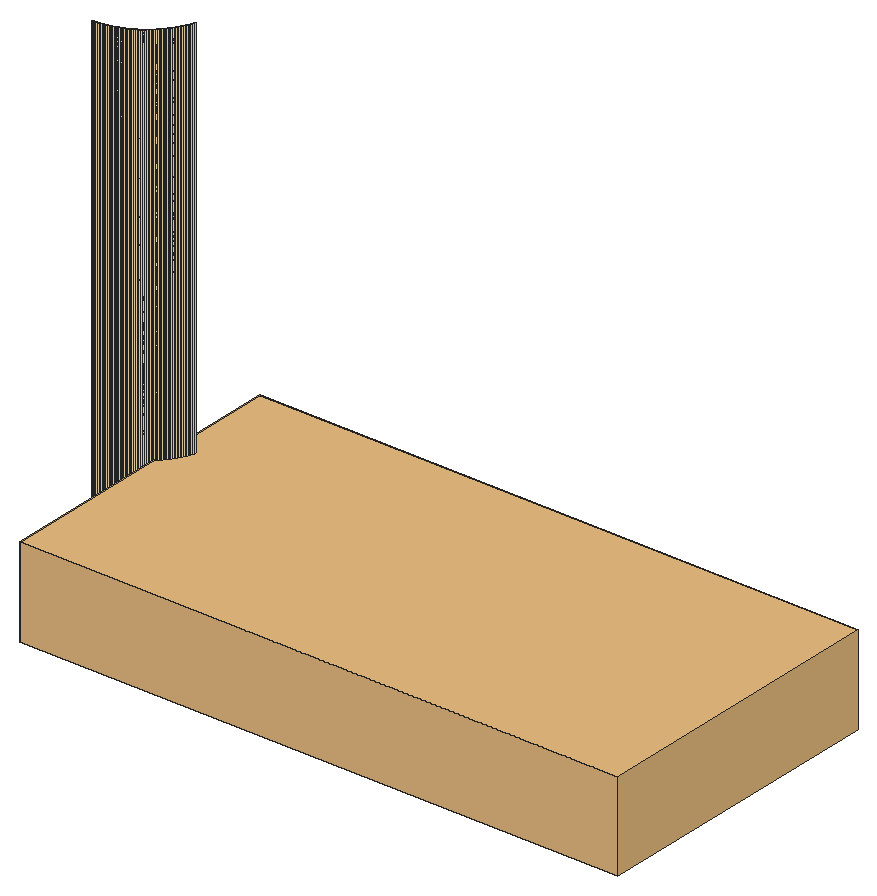
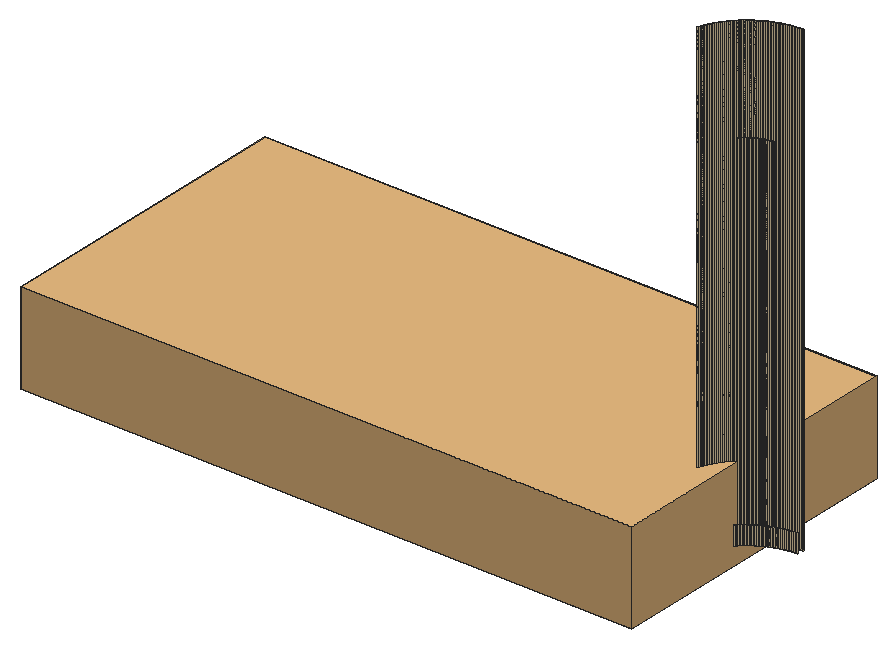
# SketchUp Ruby script. Lengths in inches.
U = 1.inch
M = Sketchup.active_model
def pt(a) = Geom::Point3d.new(a.map { |v| v * U })
def face(e, loops, mat)
  f = e.add_face(loops[0].map { |a| pt(a) })
  loops[1..].each { |l| e.add_face(l.map { |a| pt(a) }).erase! }
  f.material = f.back_material = mat if mat
  f
end
# faces: each face lists its corners as indices into pts; further lists are holes
def faces(e, pts, list, mat = nil) = list.each { |f| face(e, (f[0].is_a?(Array) ? f : [f]).map { |l| l.map { |i| pts[i] } }, mat) }
# xy, xz, yz: faces in a plane at the given z, y or x. An outline is a flat list of corners, or four numbers for a rectangle; further outlines are holes
def ring(l) = l.size == 4 ? [[l[0], l[1]], [l[2], l[1]], [l[2], l[3]], [l[0], l[3]]] : l.each_slice(2).to_a
def flat(e, list, mat, &to3) = list.each { |f| face(e, (f[0].is_a?(Array) ? f : [f]).map { |l| ring(l).map { |u, v| to3.(u, v) } }, mat) }
def xy(e, z, list, mat = nil) = flat(e, list, mat) { |x, y| [x, y, z] }
def xz(e, y, list, mat = nil) = flat(e, list, mat) { |x, z| [x, y, z] }
def yz(e, x, list, mat = nil) = flat(e, list, mat) { |y, z| [x, y, z] }
def lines(e, pts, list) = list.each { |a, b| e.add_line(pt(pts[a]), pt(pts[b])) }
# prism: a flat outline (further loops are holes) pulled along v
def prism(e, loops, v, mat = nil)
  f = face(e, loops, mat); d = Geom::Vector3d.new(v.map { |x| x * U })
  f.pushpull(f.normal.samedirection?(d) ? d.length : -d.length)
end
def box(e, o, s, mat = nil) = prism(e, [[o, [o[0] + s[0], o[1], o[2]], [o[0] + s[0], o[1] + s[1], o[2]], [o[0], o[1] + s[1], o[2]]]], [0, 0, s[2]], mat)
def at(x, y, z, deg = 0) = Geom::Transformation.translation(pt([x, y, z])) * Geom::Transformation.rotation(ORIGIN, Z_AXIS, deg.degrees)
def axes(o, x, y, z) = Geom::Transformation.new([*x, 0, *y, 0, *z, 0, *pt(o).to_a, 1])
def part(name) = M.definitions.add(name)
# library, detail: a bought-in or finely detailed component or shape, given as its bounding box
def library(name, o, s) = part(name).tap { |d| box(d.entities, o, s) }
def detail(e, o, s) = box(e.add_group.entities, o, s)
def put(e, d, t, mat = nil) = e.add_instance(d, t).tap { |i| i.material = mat if mat }
def group(e, t, mat = nil) = e.add_group.tap { |g| g.transformation = t; g.material = mat if mat }.entities
root = M.entities
M.materials.add("1026 AP 7946 SUNNY SIDE UP").color = [254, 231, 186]
c1 = library("Group\#15",[-2,-2,-6.18],[196,101,30.18])
xz(root,215.01,[[177.5,120,177.75,274]],"1026 AP 7946 SUNNY SIDE UP")
xz(root,227.02,[[177.63,132,177.75,246]],"1026 AP 7946 SUNNY SIDE UP")
p = [[178.01,215.02,120],[178.01,215.02,274],[177.75,215.01,274],[177.75,215.01,120],[178.26,215.03,120],[178.26,215.03,274],
  [178.51,215.05,120],[178.51,215.05,274],[178.76,215.0625,120],[178.76,215.0625,274],[179.01,215.08,120],[179.01,215.08,274],
  [179.26,215.11,120],[179.26,215.11,274],[179.51,215.13,120],[179.51,215.13,274],[179.76,215.16,120],[179.76,215.16,274],
  [180.01,215.1875,120],[180.01,215.1875,274],[180.26,215.22,120],[180.26,215.22,274],[180.51,215.26,120],[180.51,215.26,274],
  [180.75,215.3,120],[180.75,215.3,274],[181,215.34,120],[181,215.34,274],[181.25,215.38,120],[181.25,215.38,274],
  [181.5,215.43,120],[181.5,215.43,274],[181.74,215.47,120],[181.74,215.47,274],[181.99,215.52,120],[181.99,215.52,274],
  [182.24,215.58,120],[182.24,215.58,274],[182.48,215.63,120],[182.48,215.63,274],[182.72,215.69,120],[182.72,215.69,274],
  [182.97,215.75,120],[182.97,215.75,274],[183.21,215.82,120],[183.21,215.82,274],[183.45,215.88,120],[183.45,215.88,274],
  [183.7,215.95,120],[183.7,215.95,274],[183.9375,216.02,120],[183.9375,216.02,274],[184.18,216.1,120],[184.18,216.1,274],
  [184.42,216.17,120],[184.42,216.17,274],[184.66,216.25,120],[184.66,216.25,274],[184.89,216.33,120],[184.89,216.33,274],
  [185.13,216.42,120],[185.13,216.42,274],[185.37,216.51,120],[185.37,216.51,274],[185.6,216.59,120],[185.6,216.59,274],
  [185.83,216.69,120],[185.83,216.69,274],[186.07,216.78,120],[186.07,216.78,274],[186.3,216.875,120],[186.3,216.875,274],
  [186.53,216.97,120],[186.53,216.97,274],[177.92,217.02,120],[177.69,217.01,120],[177.69,217.01,126],[177.92,217.02,126],
  [178.15,217.03,120],[178.15,217.03,126],[178.38,217.04,120],[178.38,217.04,126],[178.61,217.06,120],[178.61,217.06,126],
  [186.76,217.07,120],[186.76,217.07,274],[178.84,217.08,120],[178.84,217.08,126],[179.07,217.1,120],[179.07,217.1,126],
  [179.3,217.12,120],[179.3,217.12,126],[179.53,217.15,120],[179.53,217.15,126],[179.76,217.17,120],[179.76,217.17,126],
  [186.99,217.18,120],[186.99,217.18,274],[179.99,217.2,120],[179.99,217.2,126],[180.21,217.24,120],[180.21,217.24,126],
  [180.44,217.27,120],[180.44,217.27,126],[187.22,217.28,120],[187.22,217.28,274],[180.67,217.31,120],[180.67,217.31,126],
  [180.9,217.35,120],[180.9,217.35,126],[181.12,217.39,120],[181.12,217.39,126],[187.45,217.39,120],[187.45,217.39,274],
  [181.35,217.43,120],[181.35,217.43,126],[181.57,217.48,120],[181.57,217.48,126],[187.67,217.5,120],[187.67,217.5,274],
  [181.8,217.53,120],[181.8,217.53,126],[182.02,217.58,120],[182.02,217.58,126],[187.9,217.62,120],[187.9,217.62,274],
  [182.25,217.64,120],[182.25,217.64,126],[182.47,217.69,120],[182.47,217.69,126],[188.12,217.73,120],[188.12,217.73,274],
  [182.69,217.75,120],[182.69,217.75,126],[182.92,217.81,120],[182.92,217.81,126],[188.34,217.85,120],[188.34,217.85,274],
  [183.14,217.875,120],[183.14,217.875,126],[188.5625,217.97,120],[188.5625,217.97,274],[183.36,217.9375,120],[183.36,217.9375,126],
  [183.58,218.01,120],[183.58,218.01,126],[183.8,218.08,120],[183.8,218.08,126],[188.78,218.09,120],[188.78,218.09,274],
  [184.02,218.15,120],[184.02,218.15,126],[184.24,218.22,120],[184.24,218.22,126],[189,218.22,120],[189,218.22,274],
  [184.45,218.3,120],[184.45,218.3,126],[189.22,218.34,120],[189.22,218.34,274],[184.67,218.38,120],[184.67,218.38,126],
  [189.43,218.47,120],[189.43,218.47,274],[184.88,218.46,120],[184.88,218.46,126],[185.1,218.54,120],[185.1,218.54,126],
  [185.3125,218.63,120],[185.3125,218.63,126],[189.65,218.6,120],[189.65,218.6,274],[185.53,218.72,120],[185.53,218.72,126],
  [189.86,218.74,120],[189.86,218.74,274],[185.74,218.81,120],[185.74,218.81,126],[190.07,218.87,120],[190.07,218.87,274],
  [185.95,218.9,120],[185.95,218.9,126],[186.16,219,120],[186.16,219,126],[190.28,219.01,120],[190.28,219.01,274],
  [186.37,219.09,120],[186.37,219.09,126],[190.49,219.15,120],[190.49,219.15,274],[186.58,219.19,120],[186.58,219.19,126],
  [186.78,219.29,120],[186.78,219.29,126],[190.7,219.29,120],[190.7,219.29,274],[186.99,219.4,120],[186.99,219.4,126],
  [190.9,219.4375,120],[190.9,219.4375,274],[187.19,219.5,120],[187.19,219.5,126],[191.11,219.58,120],[191.11,219.58,274],
  [187.4,219.61,120],[187.4,219.61,126],[187.6,219.72,120],[187.6,219.72,126],[191.31,219.73,120],[191.31,219.73,274],
  [187.8,219.83,120],[187.8,219.83,126],[191.51,219.88,120],[191.51,219.88,274],[188,219.95,120],[188,219.95,126],
  [188.2,220.0625,120],[188.2,220.0625,126],[191.71,220.04,120],[191.71,220.04,274],[191.91,220.19,120],[191.91,220.19,274],
  [188.4,220.18,120],[188.4,220.18,126],[188.59,220.3,120],[188.59,220.3,126],[192.1,220.35,120],[192.1,220.35,274],
  [188.79,220.42,120],[188.79,220.42,126],[192.3,220.51,120],[192.3,220.51,274],[188.98,220.55,120],[188.98,220.55,126],
  [189.17,220.68,120],[189.17,220.68,126],[192.49,220.67,120],[192.49,220.67,274],[189.37,220.8,120],[189.37,220.8,126],
  [192.68,220.83,120],[192.68,220.83,274],[189.56,220.93,120],[189.56,220.93,126],[192.87,221,120],[192.87,221,274],
  [189.74,221.07,120],[189.74,221.07,126],[193.06,221.16,120],[193.06,221.16,274],[189.93,221.2,120],[189.93,221.2,126],
  [190.12,221.34,120],[190.12,221.34,126],[193.25,221.33,120],[193.25,221.33,274],[190.3,221.48,120],[190.3,221.48,126],
  [193.43,221.5,120],[193.43,221.5,274],[190.48,221.62,120],[190.48,221.62,126],[193.61,221.68,120],[193.61,221.68,274],
  [190.67,221.76,120],[190.67,221.76,126],[193.79,221.85,120],[193.79,221.85,274],[190.85,221.9,120],[190.85,221.9,126],
  [191.02,222.05,120],[191.02,222.05,126],[193.97,222.03,120],[193.97,222.03,274],[191.2,222.2,120],[191.2,222.2,126],
  [194.15,222.21,120],[194.15,222.21,274],[191.375,222.35,120],[191.375,222.35,126],[194.32,222.39,120],[194.32,222.39,274],
  [191.55,222.5,120],[191.55,222.5,126],[194.5,222.57,120],[194.5,222.57,274],[191.72,222.65,120],[191.72,222.65,126],
  [194.67,222.75,120],[194.67,222.75,274],[191.89,222.81,120],[191.89,222.81,126],[192.06,222.96,120],[192.06,222.96,126],
  [194.84,222.94,120],[194.84,222.94,274],[195,223.13,120],[195,223.13,274],[192.23,223.12,120],[192.23,223.12,126],
  [192.39,223.28,120],[192.39,223.28,126],[195.17,223.32,120],[195.17,223.32,274],[192.56,223.44,120],[192.56,223.44,126],
  [195.33,223.51,120],[195.33,223.51,274],[192.72,223.61,120],[192.72,223.61,126],[195.49,223.7,120],[195.49,223.7,274],
  [192.88,223.77,120],[192.88,223.77,126],[195.65,223.9,120],[195.65,223.9,274],[193.04,223.94,120],[193.04,223.94,126],
  [193.19,224.11,120],[193.19,224.11,126],[195.81,224.09,120],[195.81,224.09,274],[193.35,224.28,120],[193.35,224.28,126],
  [195.96,224.29,120],[195.96,224.29,274],[193.5,224.45,120],[193.5,224.45,126],[196.12,224.49,120],[196.12,224.49,274],
  [193.65,224.625,120],[193.65,224.625,126],[196.27,224.69,120],[196.27,224.69,274],[193.8,224.8,120],[193.8,224.8,126],
  [196.42,224.89,120],[196.42,224.89,274],[193.95,224.98,120],[193.95,224.98,126],[196.5625,225.1,120],[196.5625,225.1,274],
  [194.1,225.15,120],[194.1,225.15,126],[196.71,225.3,120],[196.71,225.3,274],[194.24,225.33,120],[194.24,225.33,126],
  [194.38,225.52,120],[194.38,225.52,126],[196.85,225.51,120],[196.85,225.51,274],[194.52,225.7,120],[194.52,225.7,126],
  [196.99,225.72,120],[196.99,225.72,274],[194.66,225.88,120],[194.66,225.88,126],[197.13,225.93,120],[197.13,225.93,274],
  [194.8,226.07,120],[194.8,226.07,126],[197.26,226.14,120],[197.26,226.14,274],[194.93,226.26,120],[194.93,226.26,126],
  [197.4,226.35,120],[197.4,226.35,274],[195.07,226.44,120],[195.07,226.44,126],[195.2,226.63,120],[195.2,226.63,126],
  [197.53,226.57,120],[197.53,226.57,274],[195.32,226.83,120],[195.32,226.83,126],[197.66,226.78,120],[197.66,226.78,274],
  [195.45,227.02,120],[195.45,227.02,126],[197.78,227,120],[197.78,227,274],[195.58,227.21,120],[195.58,227.21,126],
  [197.91,227.22,120],[197.91,227.22,274],[195.7,227.41,120],[195.7,227.41,126],[198.03,227.4375,120],[198.03,227.4375,274],
  [195.82,227.6,120],[195.82,227.6,126],[198.15,227.66,120],[198.15,227.66,274],[195.9375,227.8,120],[195.9375,227.8,126],
  [198.27,227.88,120],[198.27,227.88,274],[196.05,228,120],[196.05,228,126],[198.38,228.1,120],[198.38,228.1,274],
  [196.17,228.2,120],[196.17,228.2,126],[198.5,228.33,120],[198.5,228.33,274],[196.28,228.4,120],[196.28,228.4,126],
  [198.61,228.55,120],[198.61,228.55,274],[196.39,228.6,120],[196.39,228.6,126],[196.5,228.81,120],[196.5,228.81,126],
  [198.72,228.78,120],[198.72,228.78,274],[196.6,229.01,120],[196.6,229.01,126],[198.82,229.01,120],[198.82,229.01,274],
  [196.71,229.22,120],[196.71,229.22,126],[198.93,229.24,120],[198.93,229.24,274],[196.81,229.42,120],[196.81,229.42,126],
  [199.03,229.47,120],[199.03,229.47,274],[196.91,229.63,120],[196.91,229.63,126],[199.125,229.7,120],[199.125,229.7,274],
  [197,229.84,120],[197,229.84,126],[199.22,229.93,120],[199.22,229.93,274],[197.1,230.05,120],[197.1,230.05,126],
  [199.31,230.17,120],[199.31,230.17,274],[197.19,230.26,120],[197.19,230.26,126],[199.41,230.4,120],[199.41,230.4,274],
  [197.28,230.47,120],[197.28,230.47,126],[199.49,230.63,120],[199.49,230.63,274],[197.37,230.6875,120],[197.37,230.6875,126],
  [199.58,230.87,120],[199.58,230.87,274],[197.46,230.9,120],[197.46,230.9,126],[197.54,231.12,120],[197.54,231.12,126],
  [199.67,231.11,120],[199.67,231.11,274],[177.75,227.02,132],[177.75,227.02,246],[177.88,227.03,246],[177.88,227.03,132],
  [178,227.04,246],[178,227.04,132],[178.13,227.05,246],[178.13,227.05,132],[178.25,227.07,246],[178.25,227.07,132],
  [178.38,227.08,246],[178.38,227.08,132],[178.5,227.09,246],[178.5,227.09,132],[178.63,227.11,246],[178.63,227.11,132],
  [178.75,227.13,246],[178.75,227.13,132],[178.88,227.15,246],[178.88,227.15,132],[179,227.17,246],[179,227.17,132],
  [179.125,227.19,246],[179.125,227.19,132],[179.25,227.21,246],[179.25,227.21,132],[179.37,227.24,246],[179.37,227.24,132],
  [179.49,227.26,246],[179.49,227.26,132],[179.62,227.29,246],[179.62,227.29,132],[179.74,227.32,246],[179.74,227.32,132],
  [179.86,227.35,246],[179.86,227.35,132],[179.98,227.38,246],[179.98,227.38,132],[180.11,227.41,246],[180.11,227.41,132],
  [180.23,227.44,246],[180.23,227.44,132],[180.35,227.48,246],[180.35,227.48,132],[180.47,227.51,246],[180.47,227.51,132],
  [180.59,227.55,246],[180.59,227.55,132],[180.71,227.59,246],[180.71,227.59,132],[180.83,227.625,246],[180.83,227.625,132],
  [180.95,227.67,246],[180.95,227.67,132],[181.06,227.71,246],[181.06,227.71,132],[181.18,227.75,246],[181.18,227.75,132],
  [181.3,227.8,246],[181.3,227.8,132],[181.42,227.84,246],[181.42,227.84,132],[181.53,227.89,246],[181.53,227.89,132],
  [181.65,227.9375,246],[181.65,227.9375,132],[181.77,227.99,246],[181.77,227.99,132],[181.88,228.04,246],[181.88,228.04,132],
  [182,228.09,246],[182,228.09,132],[182.11,228.14,246],[182.11,228.14,132],[182.22,228.2,246],[182.22,228.2,132],
  [182.34,228.25,246],[182.34,228.25,132],[182.45,228.31,246],[182.45,228.31,132],[182.56,228.37,246],[182.56,228.37,132],
  [182.67,228.42,246],[182.67,228.42,132],[182.78,228.48,246],[182.78,228.48,132],[182.89,228.55,246],[182.89,228.55,132],
  [183,228.61,246],[183,228.61,132],[183.11,228.67,246],[183.11,228.67,132],[183.22,228.74,246],[183.22,228.74,132],
  [183.32,228.8,246],[183.32,228.8,132],[183.43,228.87,246],[183.43,228.87,132],[183.54,228.9375,246],[183.54,228.9375,132],
  [183.64,229,246],[183.64,229,132],[183.75,229.08,246],[183.75,229.08,132],[183.85,229.15,246],[183.85,229.15,132],
  [183.95,229.22,246],[183.95,229.22,132],[184.05,229.29,246],[184.05,229.29,132],[184.15,229.37,246],[184.15,229.37,132],
  [184.26,229.44,246],[184.26,229.44,132],[184.35,229.52,246],[184.35,229.52,132],[184.45,229.6,246],[184.45,229.6,132],
  [184.55,229.67,246],[184.55,229.67,132],[184.65,229.75,246],[184.65,229.75,132],[184.75,229.83,246],[184.75,229.83,132],
  [184.84,229.92,246],[184.84,229.92,132],[184.9375,230,246],[184.9375,230,132],[185.03,230.08,246],[185.03,230.08,132],
  [185.12,230.17,246],[185.12,230.17,132],[185.21,230.25,246],[185.21,230.25,132],[185.31,230.34,246],[185.31,230.34,132],
  [185.4,230.43,246],[185.4,230.43,132],[185.49,230.51,246],[185.49,230.51,132],[185.57,230.6,246],[185.57,230.6,132],
  [185.66,230.69,246],[185.66,230.69,132],[185.75,230.79,246],[185.75,230.79,132],[185.83,230.88,246],[185.83,230.88,132],
  [185.92,230.97,246],[185.92,230.97,132],[186,231.0625,246],[186,231.0625,132],[186.08,231.16,246],[186.08,231.16,132],
  [186.17,231.25,246],[186.17,231.25,132]]
faces(root,p,[[0,1,2,3],[4,5,1,0],[6,7,5,4],[8,9,7,6],[10,11,9,8],[12,13,11,10],[14,15,13,12],[16,17,15,14],
  [18,19,17,16],[20,21,19,18],[22,23,21,20],[24,25,23,22],[26,27,25,24],[28,29,27,26],[30,31,29,28],[32,33,31,30],
  [34,35,33,32],[36,37,35,34],[38,39,37,36],[40,41,39,38],[42,43,41,40],[44,45,43,42],[46,47,45,44],[48,49,47,46],
  [50,51,49,48],[52,53,51,50],[54,55,53,52],[56,57,55,54],[58,59,57,56],[60,61,59,58],[62,63,61,60],[64,65,63,62],
  [66,67,65,64],[68,69,67,66],[70,71,69,68],[72,73,71,70],[74,75,76,77],[78,74,77,79],[80,78,79,81],[82,80,81,83],
  [84,85,73,72],[86,82,83,87],[88,86,87,89],[90,88,89,91],[92,90,91,93],[94,92,93,95],[96,97,85,84],[98,94,95,99],
  [100,98,99,101],[102,100,101,103],[104,105,97,96],[106,102,103,107],[108,106,107,109],[110,108,109,111],[112,113,105,104],[114,110,111,115],
  [116,114,115,117],[118,119,113,112],[120,116,117,121],[122,120,121,123],[124,125,119,118],[126,122,123,127],[128,126,127,129],[130,131,125,124],
  [132,128,129,133],[134,132,133,135],[136,137,131,130],[138,134,135,139],[140,141,137,136],[142,138,139,143],[144,142,143,145],[146,144,145,147],
  [148,149,141,140],[150,146,147,151],[152,150,151,153],[154,155,149,148],[156,152,153,157],[158,159,155,154],[160,156,157,161],[162,163,159,158],
  [164,160,161,165],[166,164,165,167],[168,166,167,169],[170,171,163,162],[172,168,169,173],[174,175,171,170],[176,172,173,177],[178,179,175,174],
  [180,176,177,181],[182,180,181,183],[184,185,179,178],[186,182,183,187],[188,189,185,184],[190,186,187,191],[192,190,191,193],[194,195,189,188],
  [196,192,193,197],[198,199,195,194],[200,196,197,201],[202,203,199,198],[204,200,201,205],[206,204,205,207],[208,209,203,202],[210,206,207,211],
  [212,213,209,208],[214,210,211,215],[216,214,215,217],[218,219,213,212],[220,221,219,218],[222,216,217,223],[224,222,223,225],[226,227,221,220],
  [228,224,225,229],[230,231,227,226],[232,228,229,233],[234,232,233,235],[236,237,231,230],[238,234,235,239],[240,241,237,236],[242,238,239,243],
  [244,245,241,240],[246,242,243,247],[248,249,245,244],[250,246,247,251],[252,250,251,253],[254,255,249,248],[256,252,253,257],[258,259,255,254],
  [260,256,257,261],[262,263,259,258],[264,260,261,265],[266,267,263,262],[268,264,265,269],[270,268,269,271],[272,273,267,266],[274,270,271,275],
  [276,277,273,272],[278,274,275,279],[280,281,277,276],[282,278,279,283],[284,285,281,280],[286,282,283,287],[288,289,285,284],[290,286,287,291],
  [292,290,291,293],[294,295,289,288],[296,297,295,294],[298,292,293,299],[300,298,299,301],[302,303,297,296],[304,300,301,305],[306,307,303,302],
  [308,304,305,309],[310,311,307,306],[312,308,309,313],[314,315,311,310],[316,312,313,317],[318,316,317,319],[320,321,315,314],[322,318,319,323],
  [324,325,321,320],[326,322,323,327],[328,329,325,324],[330,326,327,331],[332,333,329,328],[334,330,331,335],[336,337,333,332],[338,334,335,339],
  [340,341,337,336],[342,338,339,343],[344,345,341,340],[346,342,343,347],[348,346,347,349],[350,351,345,344],[352,348,349,353],[354,355,351,350],
  [356,352,353,357],[358,359,355,354],[360,356,357,361],[362,363,359,358],[364,360,361,365],[366,367,363,362],[368,364,365,369],[370,368,369,371],
  [372,373,367,366],[374,370,371,375],[376,377,373,372],[378,374,375,379],[380,381,377,376],[382,378,379,383],[384,385,381,380],[386,382,383,387],
  [388,389,385,384],[390,386,387,391],[392,393,389,388],[394,390,391,395],[396,397,393,392],[398,394,395,399],[400,401,397,396],[402,398,399,403],
  [404,405,401,400],[406,402,403,407],[408,409,405,404],[410,406,407,411],[412,410,411,413],[414,415,409,408],[416,412,413,417],[418,419,415,414],
  [420,416,417,421],[422,423,419,418],[424,420,421,425],[426,427,423,422],[428,424,425,429],[430,431,427,426],[432,428,429,433],[434,435,431,430],
  [436,432,433,437],[438,439,435,434],[440,436,437,441],[442,443,439,438],[444,440,441,445],[446,447,443,442],[448,444,445,449],[450,451,447,446],
  [452,448,449,453],[454,452,453,455],[456,457,451,450],[458,459,460,461],[461,460,462,463],[463,462,464,465],[465,464,466,467],[467,466,468,469],
  [469,468,470,471],[471,470,472,473],[473,472,474,475],[475,474,476,477],[477,476,478,479],[479,478,480,481],[481,480,482,483],[483,482,484,485],
  [485,484,486,487],[487,486,488,489],[489,488,490,491],[491,490,492,493],[493,492,494,495],[495,494,496,497],[497,496,498,499],[499,498,500,501],
  [501,500,502,503],[503,502,504,505],[505,504,506,507],[507,506,508,509],[509,508,510,511],[511,510,512,513],[513,512,514,515],[515,514,516,517],
  [517,516,518,519],[519,518,520,521],[521,520,522,523],[523,522,524,525],[525,524,526,527],[527,526,528,529],[529,528,530,531],[531,530,532,533],
  [533,532,534,535],[535,534,536,537],[537,536,538,539],[539,538,540,541],[541,540,542,543],[543,542,544,545],[545,544,546,547],[547,546,548,549],
  [549,548,550,551],[551,550,552,553],[553,552,554,555],[555,554,556,557],[557,556,558,559],[559,558,560,561],[561,560,562,563],[563,562,564,565],
  [565,564,566,567],[567,566,568,569],[569,568,570,571],[571,570,572,573],[573,572,574,575],[575,574,576,577],[577,576,578,579],[579,578,580,581],
  [581,580,582,583],[583,582,584,585],[585,584,586,587],[587,586,588,589],[589,588,590,591],[591,590,592,593],[593,592,594,595],[595,594,596,597],
  [597,596,598,599],[599,598,600,601],[601,600,602,603],[603,602,604,605],[605,604,606,607],[607,606,608,609],[609,608,610,611],[611,610,612,613]],"1026 AP 7946 SUNNY SIDE UP")
put(root,c1,axes([195.49,167,120],[1.02842,0,0],[0,1,0],[0,0,1]),"1026 AP 7946 SUNNY SIDE UP")
